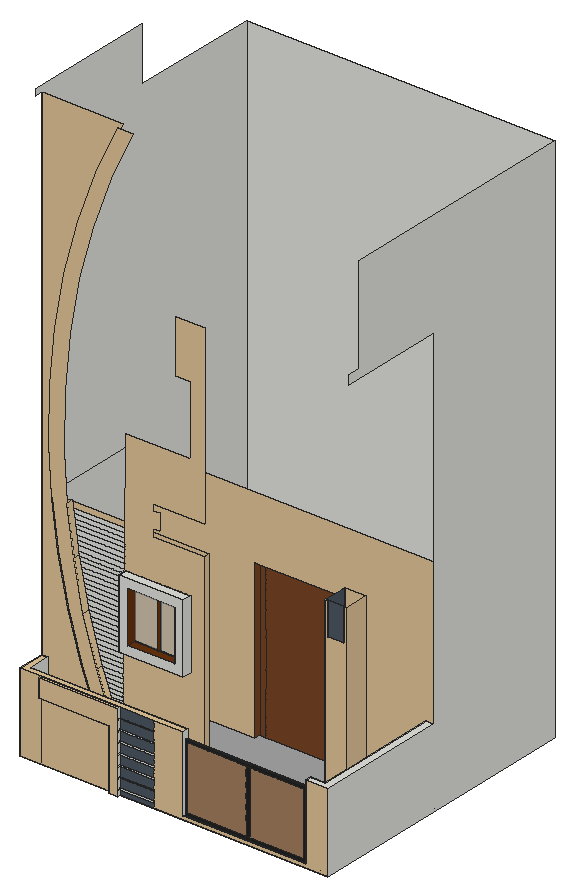
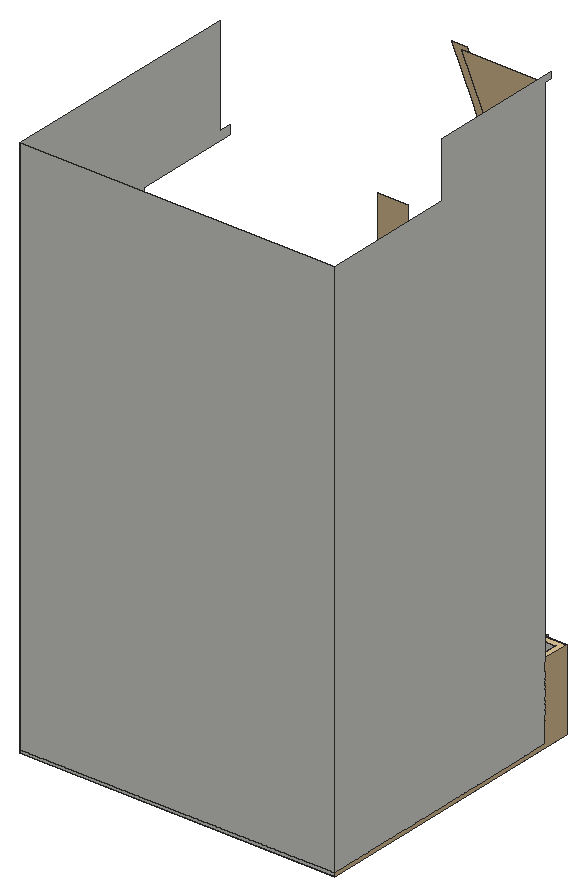
# SketchUp Ruby script. Lengths in inches.
U = 1.inch
M = Sketchup.active_model
def pt(a) = Geom::Point3d.new(a.map { |v| v * U })
def face(e, loops, mat)
  f = e.add_face(loops[0].map { |a| pt(a) })
  loops[1..].each { |l| e.add_face(l.map { |a| pt(a) }).erase! }
  f.material = f.back_material = mat if mat
  f
end
# faces: each face lists its corners as indices into pts; further lists are holes
def faces(e, pts, list, mat = nil) = list.each { |f| face(e, (f[0].is_a?(Array) ? f : [f]).map { |l| l.map { |i| pts[i] } }, mat) }
# xy, xz, yz: faces in a plane at the given z, y or x. An outline is a flat list of corners, or four numbers for a rectangle; further outlines are holes
def ring(l) = l.size == 4 ? [[l[0], l[1]], [l[2], l[1]], [l[2], l[3]], [l[0], l[3]]] : l.each_slice(2).to_a
def flat(e, list, mat, &to3) = list.each { |f| face(e, (f[0].is_a?(Array) ? f : [f]).map { |l| ring(l).map { |u, v| to3.(u, v) } }, mat) }
def xy(e, z, list, mat = nil) = flat(e, list, mat) { |x, y| [x, y, z] }
def xz(e, y, list, mat = nil) = flat(e, list, mat) { |x, z| [x, y, z] }
def yz(e, x, list, mat = nil) = flat(e, list, mat) { |y, z| [x, y, z] }
def lines(e, pts, list) = list.each { |a, b| e.add_line(pt(pts[a]), pt(pts[b])) }
# prism: a flat outline (further loops are holes) pulled along v
def prism(e, loops, v, mat = nil)
  f = face(e, loops, mat); d = Geom::Vector3d.new(v.map { |x| x * U })
  f.pushpull(f.normal.samedirection?(d) ? d.length : -d.length)
end
def box(e, o, s, mat = nil) = prism(e, [[o, [o[0] + s[0], o[1], o[2]], [o[0] + s[0], o[1] + s[1], o[2]], [o[0], o[1] + s[1], o[2]]]], [0, 0, s[2]], mat)
def at(x, y, z, deg = 0) = Geom::Transformation.translation(pt([x, y, z])) * Geom::Transformation.rotation(ORIGIN, Z_AXIS, deg.degrees)
def axes(o, x, y, z) = Geom::Transformation.new([*x, 0, *y, 0, *z, 0, *pt(o).to_a, 1])
def part(name) = M.definitions.add(name)
# library, detail: a bought-in or finely detailed component or shape, given as its bounding box
def library(name, o, s) = part(name).tap { |d| box(d.entities, o, s) }
def detail(e, o, s) = box(e.add_group.entities, o, s)
def put(e, d, t, mat = nil) = e.add_instance(d, t).tap { |i| i.material = mat if mat }
def group(e, t, mat = nil) = e.add_group.tap { |g| g.transformation = t; g.material = mat if mat }.entities
root = M.entities
M.materials.add("[0033_NavajoWhite]").color = [226, 197, 153]
M.materials.add("[0043_SaddleBrown]").color = [104, 51, 14]
M.materials.add("[0066_Honeydew]").color = [240, 255, 240]
M.materials.add("[0111_SlateGray]").color = [77, 88, 99]
M.materials.add("[0136_Charcoal]").color = [35, 35, 35]
M.materials.add("[Cladding Siding Tan]").color = [162, 126, 95]
M.materials.add("[Stone Vein Gray]").color = [166, 165, 165]
M.materials.add("[Translucent Glass Gray]").color = [193, 193, 193]
M.materials["[Translucent Glass Gray]"].alpha = 0.5
M.materials.add("[Wood Veneer 01]").color = [120, 70, 37]
xy(root,0,[[362.26,0,398.26,12],[0,12,1224,1138.125]])
xy(root,12,[[648,12,1135.51,18.9],[648,24,1135.51,24,1135.51,36,1193.3125,36,1193.3125,142.125,648,142.125],[24,36,648,36,648,118.125,384,118.125,384,91.125,324,91.125,324,118.125,24,118.125],[324,91.125,324,118.125,0,118.125,0,538.125,24,538.125,24,142.125,648,142.125,648,118.125,384,118.125,384,91.125]])
xy(root,12,[[24,142.125,1108.625,142.125,1108.625,239.75,1193.3125,239.75,1193.3125,538.125,841.41,538.125,841.41,562.125,514.34,562.125,514.34,538.125,24,538.125]],"[Stone Vein Gray]")
xy(root,240,[[84,0,362.26,12]])
xy(root,285.11,[[648,18.9,1135.51,24]],"[0136_Charcoal]")
xy(root,312,[[1135.51,12,1224,12,1224,538.125,1193.3125,538.125,1193.3125,36,1135.51,36]])
xy(root,312,[[84,0,398.26,12],[0,12,648,12,648,36,24,36,24,118.125,0,118.125]],"[0033_NavajoWhite]")
xy(root,456.53,[[336.04,82.125,592.16,118.125]],"[0066_Honeydew]")
xy(root,491.21,[[370.71,82.125,557.49,118.125]],"[0043_SaddleBrown]")
xy(root,635.75,[[514.34,538.125,841.41,562.125]],"[Wood Veneer 01]")
xy(root,695.92,[[390.09,93.91,387.75,94.09,385.53,94.87,383.59,96.19,382.0625,97.97,381.04,100.09,380.61,102.4,380.78,104.74,381.56,106.96,382.88,108.9,384.67,110.43,386.78,111.45,389.09,111.89,391.43,111.71,393.65,110.93,395.59,109.61,397.125,107.83,398.14,105.71,398.58,103.4,398.4,101.06,397.625,98.84,396.3,96.9,394.52,95.37,392.4,94.35],[463.59,93.91,461.25,94.09,459.03,94.87,457.09,96.19,455.5625,97.97,454.54,100.09,454.11,102.4,454.28,104.74,455.06,106.96,456.38,108.9,458.17,110.43,460.28,111.45,462.59,111.89,464.1,111.77,464.93,111.71,467.15,110.93,469.09,109.61,470.625,107.83,471.64,105.71,472.08,103.4,471.9,101.06,471.125,98.84,469.8,96.9,468.02,95.37,465.9,94.35,464.1,94.01],[534.78,93.91,532.4375,94.09,530.22,94.87,528.28,96.19,526.75,97.97,525.73,100.09,525.29,102.4,525.47,104.74,526.25,106.96,527.57,108.9,529.35,110.43,531.47,111.45,533.78,111.89,535.29,111.77,536.12,111.71,538.34,110.93,540.28,109.61,541.8125,107.83,542.83,105.71,543.27,103.4,543.09,101.06,542.3125,98.84,540.99,96.9,539.21,95.37,537.09,94.35,535.29,94.01]])
xy(root,695.92,[[[370.71,82.125,557.49,118.125],[390.09,93.91,392.4,94.35,394.52,95.37,396.3,96.9,397.625,98.84,398.4,101.06,398.58,103.4,398.14,105.71,397.125,107.83,395.59,109.61,393.65,110.93,391.43,111.71,389.09,111.89,386.78,111.45,384.67,110.43,382.88,108.9,381.56,106.96,380.78,104.74,380.61,102.4,381.04,100.09,382.0625,97.97,383.59,96.19,385.53,94.87,387.75,94.09],[534.78,93.91,535.29,94.01,537.09,94.35,539.21,95.37,540.99,96.9,542.3125,98.84,543.09,101.06,543.27,103.4,542.83,105.71,541.8125,107.83,540.28,109.61,538.34,110.93,536.12,111.71,535.29,111.77,533.78,111.89,531.47,111.45,529.35,110.43,527.57,108.9,526.25,106.96,525.47,104.74,525.29,102.4,525.73,100.09,526.75,97.97,528.28,96.19,530.22,94.87,532.4375,94.09],[463.59,93.91,464.1,94.01,465.9,94.35,468.02,95.37,469.8,96.9,471.125,98.84,471.9,101.06,472.08,103.4,471.64,105.71,470.625,107.83,469.09,109.61,467.15,110.93,464.93,111.71,464.1,111.77,462.59,111.89,460.28,111.45,458.17,110.43,456.38,108.9,455.06,106.96,454.28,104.74,454.11,102.4,454.54,100.09,455.5625,97.97,457.09,96.19,459.03,94.87,461.25,94.09]]],"[0043_SaddleBrown]")
xy(root,730.59,[[336.04,82.125,592.16,118.125]])
xy(root,759,[[1118.15,142.125,1184.28,144.125],[1108.625,146.9375,1110.625,232.4375]],"[0111_SlateGray]")
xz(root,0,[[362.26,0,398.26,0,398.26,312,84,312,84,240,362.26,240]],"[0033_NavajoWhite]")
xz(root,12,[[362.26,0,362.26,240,84,240,84,312,398.26,312,398.26,0],[398.26,18,531.89,24],[398.26,60,531.89,66],[398.26,102,531.89,108],[398.26,144,531.89,150],
  [398.26,186,531.89,192],[398.26,228,531.89,234],[398.26,270,531.89,276]])
xz(root,12,[[0,0,84,312],[84,0,362.26,240],[531.89,0,1224,0,1224,312,1135.51,312,1135.51,12,648,12,648,312,531.89,312]],"[0033_NavajoWhite]")
xz(root,12,[[398.26,0,531.89,18],[398.26,24,531.89,60],[398.26,66,531.89,102],[398.26,108,531.89,144],[398.26,150,531.89,186],
  [398.26,192,531.89,228],[398.26,234,531.89,270],[398.26,276,531.89,312]],"[0111_SlateGray]")
xz(root,18.9,[[648,12,891.75,12,891.75,24,660,24,660,273.11,891.75,273.11,891.75,285.11,648,285.11],[891.75,12,906.3,24],[906.3,12,1135.51,12,1135.51,285.11,906.3,285.11,906.3,273.11,1123.51,273.11,1123.51,24,906.3,24],[891.75,24,906.3,273.11],[891.75,273.11,906.3,285.11]],"[0136_Charcoal]")
xz(root,18.9,[[660,24,891.75,273.11],[906.3,24,1123.51,273.11]],"[Cladding Siding Tan]")
xz(root,24,[[648,12,1135.51,285.11]])
xz(root,36,[[24,12,648,312],[1135.51,12,1193.3125,312]])
xz(root,82.125,[[[336.04,456.53,592.16,730.59],[370.71,491.21,557.49,695.92]]])
xz(root,91.125,[[324,12,384,12,305.79,182.19,240.25,357.65,187.73,537.4375,148.51,720.59,122.81,906.12,110.76,1093.03,113.6,1303.95,133.83,1513.92,171.29,1721.51,225.74,1925.31,296.81,2123.92,384,2316,324,2316,236.81,2123.92,165.74,1925.31,111.29,1721.51,73.83,1513.92,53.6,1303.95,50.76,1093.03,62.81,906.12,88.51,720.59,127.73,537.4375,180.25,357.65,245.79,182.19]],"[0033_NavajoWhite]")
xz(root,118.125,[[0,12,24,312],[321.59,147.81,321.96,174.8125,309.18,174.8125],[309.18,174.8125,321.96,174.8125,322.02,179.26,322.14,188.26,303.43,188.51,305.79,182.19],[322.14,188.26,322.26,197.26,322.33,202.16,298.33,202.16,303.43,188.51],[298.33,202.16,322.33,202.16,322.49,214.25,293.67,214.64],
  [322.49,214.25,322.72,231.25,287.47,231.25,293.67,214.64],[287.47,231.25,322.72,231.25,322.93,246.71,281.6875,246.71],[281.6875,246.71,322.93,246.71,323.12,260.8,276.43,260.8],[276.43,260.8,323.12,260.8,323.3,274.33,271.37,274.33],[271.37,274.33,323.3,274.33,323.52,290.42,265.36,290.42],
  [265.36,290.42,323.52,290.42,323.73,305.88,259.59,305.88],[259.59,305.88,323.73,305.88,323.94,321.78,253.65,321.78],[253.65,321.78,323.94,321.78,324.18,339.78,246.93,339.78],[246.93,339.78,324.18,339.78,324.43,357.78,240.25,357.65],[240.25,357.65,324.43,357.78,324.67,375.78,234.95,375.78],
  [234.95,375.78,324.67,375.78,324.91,393.78,229.7,393.78],[229.7,393.78,324.91,393.78,325.16,411.78,224.4375,411.78],[224.4375,411.78,325.16,411.78,325.4,429.78,219.18,429.78],[219.18,429.78,325.4,429.78,325.64,447.78,213.92,447.78],[213.92,447.78,325.64,447.78,325.89,465.78,208.66,465.78],
  [[336.04,456.53,592.16,730.59],[370.71,491.21,557.49,695.92]],[208.66,465.78,336.04,465.78,336.04,483.78,203.41,483.78],[203.41,483.78,336.04,483.78,336.04,501.78,198.15,501.78],[198.15,501.78,336.04,501.78,336.04,519.78,192.89,519.78],[192.89,519.78,336.04,519.78,336.04,537.78,187.66,537.78,187.73,537.4375],
  [187.66,537.78,336.04,537.78,336.04,555.78,183.8,555.78],[183.8,555.78,336.04,555.78,336.04,573.78,179.95,573.78],[179.95,573.78,336.04,573.78,336.04,591.78,176.09,591.78],[176.09,591.78,336.04,591.78,336.04,609.78,172.24,609.78],[172.24,609.78,336.04,609.78,336.04,627.78,168.39,627.78],
  [168.39,627.78,336.04,627.78,336.04,645.78,164.53,645.78],[164.53,645.78,336.04,645.78,336.04,663.78,160.68,663.78],[160.68,663.78,336.04,663.78,336.04,681.78,156.82,681.78],[156.82,681.78,336.04,681.78,336.04,699.78,152.97,699.78],[152.97,699.78,336.04,699.78,336.04,717.78,149.11,717.78],
  [149.11,717.78,329.29,717.78,329.53,735.78,146.41,735.78,148.51,720.59],[146.41,735.78,329.53,735.78,329.77,753.78,143.91,753.78],[143.91,753.78,329.77,753.78,330.02,771.78,141.42,771.78],[141.42,771.78,330.02,771.78,330.26,789.78,138.93,789.78],[138.93,789.78,330.26,789.78,330.5,807.78,136.43,807.78],
  [136.43,807.78,330.5,807.78,330.75,825.78,133.9375,825.78],[133.9375,825.78,330.75,825.78,330.99,843.78,131.45,843.78],[131.45,843.78,330.99,843.78,331.23,861.78,128.95,861.78],[128.95,861.78,331.23,861.78,331.48,879.78,126.46,879.78]])
xz(root,118.125,[[24,12,324,12,245.79,182.19,180.25,357.65,127.73,537.4375,88.51,720.59,62.81,906.12,50.76,1093.03,53.6,1303.95,73.83,1513.92,111.29,1721.51,165.74,1925.31,236.81,2123.92,324,2316,0,2316,0,312,24,312],[384,12,648,12,648,888,444,888,444,918,471.99,918,471.99,982.5625,444,982.5625,444,1006.5625,648,1006.5625,648,1704,534.32,1704,534.32,1491.78,592.16,1491.78,592.16,1217.72,336.04,1217.72,335.85,1203.78,335.61,1185.78,335.36,1167.78,334.88,1131.78,334.63,1113.78,333.91,1059.78,333.66,1041.78,333.18,1005.78,332.93,987.78,332.45,951.78,332.2,933.78,331.48,879.78,331.23,861.78,330.75,825.78,330.5,807.78,330.02,771.78,329.77,753.78,329.29,717.78,336.04,717.78,336.04,730.59,592.16,730.59,592.16,456.53,336.04,456.53,336.04,465.78,325.89,465.78,325.64,447.78,325.16,411.78,324.91,393.78,324.43,357.78,324.18,339.78,323.94,321.78,323.73,305.88,323.52,290.42,323.3,274.33,323.12,260.8,322.93,246.71,322.72,231.25,322.49,214.25,322.33,202.16,322.26,197.26,322.02,179.26,321.96,174.8125,321.59,147.81]],"[0033_NavajoWhite]")
xz(root,118.125,[[464.1,491.21,473.1,695.92]],"[0043_SaddleBrown]")
xz(root,118.125,[[370.71,491.21,464.1,695.92],[473.1,491.21,557.49,695.92]],"[Translucent Glass Gray]")
xz(root,142.125,[[24,12,648,888],[1108.625,12,1193.3125,12,1193.3125,888,1184.28,888,1184.28,759,1118.15,759,1118.15,888,1108.625,888]],"[0033_NavajoWhite]")
xz(root,144.125,[[1118.15,759,1184.28,888]],"[0111_SlateGray]")
xz(root,146.9375,[[1108.625,759,1110.625,888]])
xz(root,232.4375,[[1108.625,759,1110.625,888]],"[0111_SlateGray]")
xz(root,239.75,[[1108.625,12,1193.3125,888]],"[0033_NavajoWhite]")
xz(root,538.125,[[24,12,514.34,12,514.34,635.75,841.41,635.75,841.41,12,1193.3125,12,1193.3125,312,1224,312,1224,888,24,888]],"[0033_NavajoWhite]")
xz(root,562.125,[[813.99,316.13,816.32,316.44,818.49,317.34,820.36,318.77,821.79,320.63,822.6875,322.8,822.99,325.13,822.6875,327.46,821.79,329.63,820.36,331.5,818.49,332.93,816.32,333.83,813.99,334.13,811.66,333.83,809.49,332.93,807.63,331.5,806.2,329.63,805.3,327.46,804.99,325.13,805.3,322.8,806.2,320.63,807.63,318.77,809.49,317.34,811.66,316.44]])
xz(root,562.125,[[514.34,12,538.34,635.75],[538.34,12,801.97,635.75],[[801.97,12,841.41,635.75],[813.99,316.13,811.66,316.44,809.49,317.34,807.63,318.77,806.2,320.63,805.3,322.8,804.99,325.13,805.3,327.46,806.2,329.63,807.63,331.5,809.49,332.93,811.66,333.83,813.99,334.13,816.32,333.83,818.49,332.93,820.36,331.5,821.79,329.63,822.6875,327.46,822.99,325.13,822.6875,322.8,821.79,320.63,820.36,318.77,818.49,317.34,816.32,316.44]]],"[Wood Veneer 01]")
xz(root,1138.125,[[0,0,1224,12],[0,12,1224,2124]])
yz(root,0,[[118.125,12,118.125,2316,91.125,2316,91.125,2340,619,2340,619,2124,1138.125,2124,1138.125,12]])
yz(root,0,[[12,0,12,312,118.125,312,118.125,12,1138.125,12,1138.125,0]],"[0033_NavajoWhite]")
yz(root,24,[[36,12,118.125,312],[142.125,12,538.125,888]])
yz(root,84,[[0,240,12,312]],"[0033_NavajoWhite]")
yz(root,336.04,[[82.125,456.53,118.125,730.59]])
yz(root,362.26,[[0,0,12,240]],"[0033_NavajoWhite]")
yz(root,370.71,[[82.125,491.21,118.125,695.92]],"[0043_SaddleBrown]")
yz(root,398.26,[[0,0,12,18],[0,18,12,24],[0,24,12,60],[0,60,12,66],[0,66,12,102],
  [0,102,12,108],[0,108,12,144],[0,144,12,150],[0,150,12,186],[0,186,12,192],
  [0,192,12,228],[0,228,12,234],[0,234,12,270],[0,270,12,276],[0,276,12,312]])
yz(root,514.34,[[538.125,12,562.125,635.75]],"[Wood Veneer 01]")
yz(root,557.49,[[82.125,491.21,118.125,695.92]],"[0043_SaddleBrown]")
yz(root,592.16,[[82.125,456.53,118.125,730.59]])
yz(root,648,[[12,12,18.9,12,18.9,285.11,24,285.11,24,12,36,12,36,312,12,312]])
yz(root,648,[[118.125,12,142.125,888]],"[0033_NavajoWhite]")
yz(root,841.41,[[538.125,12,562.125,635.75]],"[Wood Veneer 01]")
yz(root,1108.625,[[142.125,12,142.125,888,146.9375,888,146.9375,759,232.4375,759,232.4375,888,239.75,888,239.75,12]],"[0033_NavajoWhite]")
yz(root,1110.625,[[146.9375,759,232.4375,888]],"[0111_SlateGray]")
yz(root,1118.15,[[142.125,759,144.125,888]],"[0111_SlateGray]")
yz(root,1135.51,[[12,12,12,312,36,312,36,12,24,12,24,285.11,18.9,285.11,18.9,12]])
yz(root,1184.28,[[142.125,759,144.125,888]],"[0111_SlateGray]")
yz(root,1193.3125,[[36,12,142.125,312],[142.125,12,239.75,312],[239.75,12,538.125,312]])
yz(root,1193.3125,[[142.125,312,239.75,888]],"[0033_NavajoWhite]")
yz(root,1224,[[12,0,1138.125,0,1138.125,2124,166.125,2124,166.125,1740,118.125,1740,118.125,1704,538.125,1704,538.125,312,12,312]])
p = [[245.79,118.125,182.19],[324,118.125,12],[324,91.125,12],[245.79,91.125,182.19],[309.18,118.125,174.8125],[305.79,118.125,182.19],
  [305.79,91.125,182.19],[384,91.125,12],[384,118.125,12],[321.59,118.125,147.81],[180.25,118.125,357.65],[180.25,91.125,357.65],
  [246.93,118.125,339.78],[240.25,118.125,357.65],[240.25,91.125,357.65],[303.43,118.125,188.51],[298.33,118.125,202.16],[293.67,118.125,214.64],
  [287.47,118.125,231.25],[281.6875,118.125,246.71],[276.43,118.125,260.8],[271.37,118.125,274.33],[265.36,118.125,290.42],[259.59,118.125,305.88],
  [253.65,118.125,321.78],[127.73,118.125,537.4375],[127.73,91.125,537.4375],[192.89,118.125,519.78],[187.73,118.125,537.4375],[187.73,91.125,537.4375],
  [234.95,118.125,375.78],[229.7,118.125,393.78],[224.4375,118.125,411.78],[219.18,118.125,429.78],[213.92,118.125,447.78],[208.66,118.125,465.78],
  [203.41,118.125,483.78],[198.15,118.125,501.78],[88.51,118.125,720.59],[88.51,91.125,720.59],[149.11,118.125,717.78],[148.51,118.125,720.59],
  [148.51,91.125,720.59],[187.66,118.125,537.78],[183.8,118.125,555.78],[179.95,118.125,573.78],[176.09,118.125,591.78],[172.24,118.125,609.78],
  [168.39,118.125,627.78],[164.53,118.125,645.78],[160.68,118.125,663.78],[156.82,118.125,681.78],[152.97,118.125,699.78],[62.81,118.125,906.12],
  [62.81,91.125,906.12],[123.96,118.125,897.78],[122.81,118.125,906.12],[122.81,91.125,906.12],[146.41,118.125,735.78],[143.91,118.125,753.78],
  [141.42,118.125,771.78],[138.93,118.125,789.78],[136.43,118.125,807.78],[133.9375,118.125,825.78],[131.45,118.125,843.78],[128.95,118.125,861.78],
  [126.46,118.125,879.78],[1224,538.125,12],[1193.3125,538.125,12],[1193.3125,36,12],[1193.3125,12,12],[1135.51,24,12],
  [1135.51,18.9,12]]
faces(root,p,[[0,1,2,3],[4,5,6,7,8,9],[10,0,3,11],[12,13,14,6,5,15,16,17,18,19,20,21,22,23,24],[25,10,11,26],[27,28,29,14,13,30,31,32,33,34,35,36,37],[38,25,26,39],[40,41,42,29,28,43,44,45,46,47,48,49,50,51,52],
  [53,38,39,54],[55,56,57,42,41,58,59,60,61,62,63,64,65,66]],"[0033_NavajoWhite]")
lines(root,p,[[67,68],[69,70],[71,72]])
